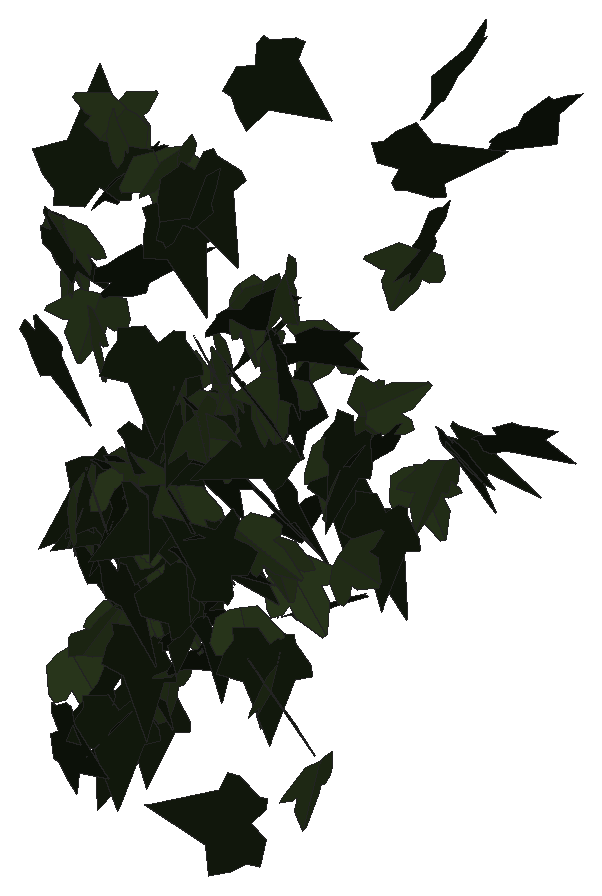
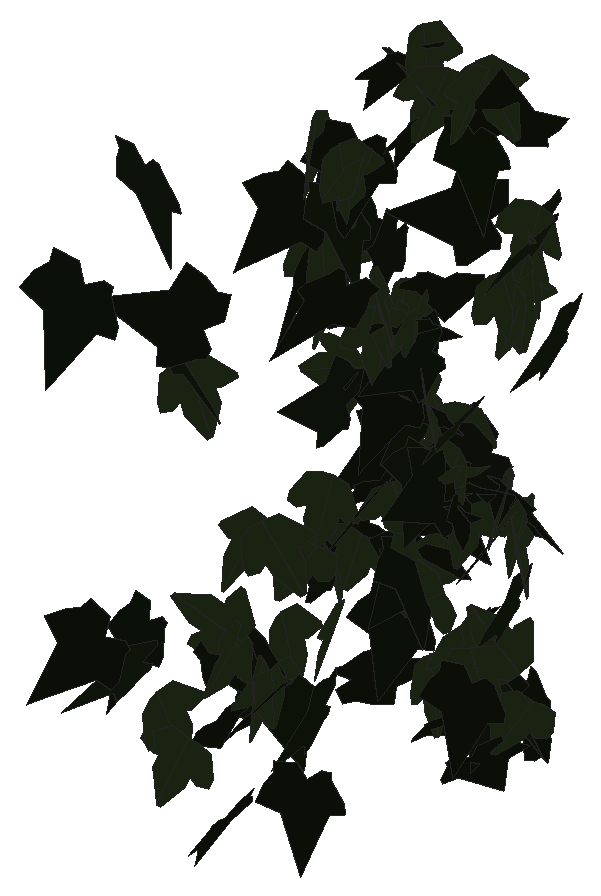
# SketchUp Ruby script. Lengths in inches.
U = 1.inch
M = Sketchup.active_model
def pt(a) = Geom::Point3d.new(a.map { |v| v * U })
def face(e, loops, mat)
  f = e.add_face(loops[0].map { |a| pt(a) })
  loops[1..].each { |l| e.add_face(l.map { |a| pt(a) }).erase! }
  f.material = f.back_material = mat if mat
  f
end
# faces: each face lists its corners as indices into pts; further lists are holes
def faces(e, pts, list, mat = nil) = list.each { |f| face(e, (f[0].is_a?(Array) ? f : [f]).map { |l| l.map { |i| pts[i] } }, mat) }
# xy, xz, yz: faces in a plane at the given z, y or x. An outline is a flat list of corners, or four numbers for a rectangle; further outlines are holes
def ring(l) = l.size == 4 ? [[l[0], l[1]], [l[2], l[1]], [l[2], l[3]], [l[0], l[3]]] : l.each_slice(2).to_a
def flat(e, list, mat, &to3) = list.each { |f| face(e, (f[0].is_a?(Array) ? f : [f]).map { |l| ring(l).map { |u, v| to3.(u, v) } }, mat) }
def xy(e, z, list, mat = nil) = flat(e, list, mat) { |x, y| [x, y, z] }
def xz(e, y, list, mat = nil) = flat(e, list, mat) { |x, z| [x, y, z] }
def yz(e, x, list, mat = nil) = flat(e, list, mat) { |y, z| [x, y, z] }
def lines(e, pts, list) = list.each { |a, b| e.add_line(pt(pts[a]), pt(pts[b])) }
# prism: a flat outline (further loops are holes) pulled along v
def prism(e, loops, v, mat = nil)
  f = face(e, loops, mat); d = Geom::Vector3d.new(v.map { |x| x * U })
  f.pushpull(f.normal.samedirection?(d) ? d.length : -d.length)
end
def box(e, o, s, mat = nil) = prism(e, [[o, [o[0] + s[0], o[1], o[2]], [o[0] + s[0], o[1] + s[1], o[2]], [o[0], o[1] + s[1], o[2]]]], [0, 0, s[2]], mat)
def at(x, y, z, deg = 0) = Geom::Transformation.translation(pt([x, y, z])) * Geom::Transformation.rotation(ORIGIN, Z_AXIS, deg.degrees)
def axes(o, x, y, z) = Geom::Transformation.new([*x, 0, *y, 0, *z, 0, *pt(o).to_a, 1])
def part(name) = M.definitions.add(name)
# library, detail: a bought-in or finely detailed component or shape, given as its bounding box
def library(name, o, s) = part(name).tap { |d| box(d.entities, o, s) }
def detail(e, o, s) = box(e.add_group.entities, o, s)
def put(e, d, t, mat = nil) = e.add_instance(d, t).tap { |i| i.material = mat if mat }
def group(e, t, mat = nil) = e.add_group.tap { |g| g.transformation = t; g.material = mat if mat }.entities
root = M.entities
M.materials.add("efeu1").color = [18, 25, 13]
M.materials.add("efeu2").color = [43, 57, 29]
c1 = part("ivyleaf_10")
p = [[0,0.5,-0.03],[-0.0625,2.02,-0.43],[-0.19,2.01,-0.46],[-0.54,1.05,-0.29],[-0.52,0.625,-0.18],[-0.83,0.76,-0.28],
  [-1.16,0.64,-0.33],[-1.15,0.33,-0.24],[-0.77,-0.39,0.02],[-0.3,-0.51,0.16],[0.04,-0.48,0.23],[-0.02,2.01,-0.4375],
  [-0.06,2.01,-0.43],[0.04,-0.49,0.23],[0.67,-0.49,0.14],[1.38,0.36,-0.2],[1.375,0.51,-0.24],[0.81,0.65,-0.19],
  [0.62,0.59,-0.15],[0.6,1.09,-0.28],[0.5,1.23,-0.31]]
faces(c1.entities,p,[[0,1,2,3,4,5,6,7,8,9,10],[11,12,0,13,14,15,16,17,18,19,20]],"efeu2")
c2 = part("ivyleaf_9")
p = [[1.54,2.16,1.25],[1.36,2.04,1.19],[-0.21,0.99,0.68],[-0.71,1.11,0.82],[-0.85,0.86,0.67],[-0.8,0.17,0.21],
  [-0.9,-0.01,0.1],[-0.67,-0.16,-0.02],[-0.08,-0.08,-0.05],[-0.03,-0.6,-0.4],[0.65,-0.88,-0.66],[0.83,-0.6,-0.49],
  [1.29,-0.42,-0.43],[1.8125,-0.07,-0.26],[1.21,0.44,0.15]]
faces(c2.entities,p,[[0,1,2,3,4,5,6,7,8,9,10,11,12,13,14]],"efeu1")
put(root,c1,axes([615.85,124.16,302.23],[-0.0433,-1.22848,-0.26768],[-0.03456,0.2689,-1.22849],[1.25683,-0.03493,-0.043]))
put(root,c2,axes([618.39,123.99,286.45],[-0.35286,0.28688,1.16377],[-0.96507,0.65147,-0.45321],[-0.71085,-1.02687,0.0376]))
put(root,c2,axes([610.3,124.6,276.83],[0.56426,-0.2794,-1.05982],[1.09365,0.22208,0.52372],[0.07223,-1.17995,0.34953]))
put(root,c2,axes([618.38,125.02,275.8125],[-0.40978,-0.84585,-0.82752],[-0.32548,-0.76138,0.93943],[-1.13768,0.52249,0.0293]))
put(root,c1,axes([619.14,124.4,287.95],[-0.46391,0.13468,-1.0838],[1.04968,-0.27011,-0.48287],[-0.30152,-1.14755,-0.01354]))
put(root,c2,axes([609.46,124.39,292.78],[0.94353,-0.81452,-0.23788],[-0.16787,0.16953,-1.24634],[0.83177,0.95818,0.0183]))
put(root,c2,axes([615.51,124.66,299.51],[0.32492,-1.16376,-0.32096],[-0.04184,0.32133,-1.20745],[1.20648,0.32456,0.04457]))
put(root,c2,axes([616.59,123.66,300.24],[0.126,0.73833,0.99377],[-0.65835,0.88592,-0.57473],[-1.04847,-0.46755,0.48031]))
put(root,c2,axes([612.74,124.89,283.93],[0.66806,-0.98934,0.14029],[0.0638,-0.12619,-1.19365],[0.9972,0.67086,-0.01762]))
put(root,c2,axes([612.64,124.95,278.25],[-0.6587,-0.72747,-0.60798],[0.50762,0.35464,-0.97431],[0.80073,-0.82326,0.11753]))
put(root,c2,axes([616.375,124.68,301.65],[0.15711,-1.07885,-0.60291],[0.15114,0.61997,-1.07],[1.22661,0.06179,0.20907]))
put(root,c1,axes([616.58,124.44,291.76],[0.01717,-1.10472,-0.47812],[0.09681,0.47789,-1.1007],[1.19984,-0.02275,0.09566]))
put(root,c2,axes([612.21,124.39,300],[-1.27822,-0.28751,0.55165],[0.53934,0.116,1.31015],[-0.31,1.38734,0.00478]))
put(root,c2,axes([614.18,125.2,293.59],[-0.5532,-0.9828,-0.49121],[0.43229,0.31091,-1.1089],[1.0101,-0.67131,0.20556]))
put(root,c2,axes([618.07,125.27,293.4],[0.61137,-0.79804,0.71074],[0.49994,-0.51012,-1.00281],[0.9445,0.78658,0.07074]))
put(root,c1,axes([615.65,124.88,288.05],[-1.10346,-0.11334,-0.39142],[0.40573,-0.20025,-1.08581],[0.03798,-1.15358,0.22694]))
put(root,c2,axes([610.11,124.48,297.16],[1.00556,-0.444,-0.55518],[-0.37168,0.49145,-1.06623],[0.60598,1.0382,0.26729]))
put(root,c2,axes([619.625,125.77,294.31],[0.03489,-0.46323,1.1072],[0.19537,-1.0907,-0.46249],[1.18419,0.19359,0.04368]))
put(root,c1,axes([614.625,124.91,301.27],[-0.93457,-0.71839,-0.39001],[0.48277,-0.00703,-1.1439],[0.65964,-1.01266,0.28462]))
put(root,c1,axes([610.46,124.86,297.15],[-1.19553,0.13285,-0.14595],[0.13754,-0.08177,-1.2011],[-0.14154,-1.20163,0.0656]))
put(root,c1,axes([612.5,125.16,302.36],[-0.94227,-0.36306,0.71281],[-0.60761,-0.39157,-1.00264],[0.52032,-1.11474,0.12003]))
put(root,c1,axes([610.3,125.01,296.03],[0.93697,-0.7882,-0.09332],[0.07276,0.22907,-1.20421],[0.79036,0.91332,0.22149]))
put(root,c2,axes([618.75,124.43,297.07],[0.38161,1.15016,-0.07246],[-0.03535,-0.06461,-1.21174],[-1.1519,0.38302,0.01318]))
put(root,c2,axes([614.35,125.82,286.55],[-0.94205,-0.44896,0.52127],[-0.34243,-0.46059,-1.01555],[0.59667,-0.97316,0.24017]))
put(root,c1,axes([611.38,125.28,294.25],[-0.80375,-0.85619,0.34099],[-0.16184,-0.31429,-1.17063],[0.90727,-0.81456,0.09326]))
put(root,c2,axes([616.9375,124.66,294.2],[0.92576,-0.09633,-0.76545],[-0.7489,0.17504,-0.92776],[0.18534,1.18841,0.0746]))
put(root,c2,axes([612.93,124.46,296.2],[0.64303,0.07724,1.11184],[0.91532,0.69576,-0.57771],[-0.63588,1.07962,0.29276]))
put(root,c2,axes([615.18,125.35,287.5625],[0.97691,-0.6502,-0.05486],[-0.05628,0.01444,-1.17335],[0.65008,0.97834,-0.01915]))
put(root,c2,axes([615.5625,125.41,284.03],[-0.99219,0.31067,0.52272],[-0.48685,0.1935,-1.0391],[-0.36433,-1.10464,-0.03501]))
put(root,c1,axes([610.91,125.32,293.71],[-0.95358,0.71123,-0.27459],[0.19567,-0.19668,-1.18895],[-0.73686,-0.97264,0.03963]))
put(root,c2,axes([616.18,124.86,286.23],[1.07533,0.33696,0.32128],[0.28206,0.17182,-1.12429],[-0.37041,1.10907,0.07657]))
put(root,c1,axes([617.2,125.3,290.77],[0.35485,0.16747,-1.12453],[-1.08733,0.39415,-0.28441],[0.33215,1.11137,0.27032]))
put(root,c2,axes([614.625,125.91,288.39],[-0.99857,-0.35101,-0.50364],[0.48678,0.13317,-1.05797],[0.37403,-1.11043,0.03232]))
put(root,c1,axes([618.46,125.64,297.09],[-0.17537,-1.20364,0.01617],[-0.01059,-0.0148,-1.21632],[1.2037,-0.17549,-0.00835]))
put(root,c1,axes([613.24,125.43,288.28],[-1.17577,-0.05594,0.1598],[-0.15831,-0.03425,-1.1768],[0.06003,-1.18609,0.02644]))
put(root,c1,axes([618.05,125.38,296.77],[-0.10181,1.22145,0.02751],[-0.00084,0.02753,-1.22568],[-1.22176,-0.1018,-0.00145]))
put(root,c2,axes([619.01,126.18,291.05],[-1.06825,-0.18471,0.47145],[-0.42037,-0.29007,-1.06616],[0.28226,-1.13105,0.19644]))
put(root,c2,axes([615.42,126.2,291.61],[-0.84454,-0.82833,-0.18309],[0.19174,0.06528,-1.17978],[0.82637,-0.86169,0.08662]))
put(root,c1,axes([619,125.65,281.72],[0.39826,-1.13674,-0.19511],[-0.06503,0.18395,-1.20449],[1.15153,0.40353,-0.00054]))
put(root,c2,axes([618.59,126.06,280.9],[0.65392,-0.73237,0.65307],[0.42924,-0.49224,-0.98181],[0.8824,0.78219,-0.00638]))
put(root,c2,axes([611.18,125.97,286.51],[-1.17568,0.08003,-0.01328],[0.01323,-0.00121,-1.1784],[-0.08004,-1.17575,0.00031]))
put(root,c1,axes([619.33,125.78,293.39],[-0.91338,-0.76601,0.12842],[-0.08853,-0.09427,-1.19197],[0.77163,-0.91753,0.01525]))
put(root,c2,axes([612.21,124.9,277.19],[0.1203,1.0288,0.50547],[0.01188,0.5071,-1.03495],[-1.14621,0.11323,0.04233]))
put(root,c1,axes([613.81,125.73,286.625],[-1.09389,0.17325,-0.34606],[0.3328,-0.10845,-1.10628],[-0.19752,-1.14219,0.05255]))
put(root,c2,axes([611.64,125.73,278.56],[-0.87687,0.74677,0.00919],[-0.02995,-0.02101,-1.15122],[-0.74622,-0.87667,0.03541]))
put(root,c1,axes([619.69,125.57,297.97],[0.33165,-1.04789,-0.51734],[0.1186,0.56517,-1.06875],[1.1626,0.24127,0.2566]))
put(root,c2,axes([612.49,126.45,280.24],[0.11928,-1.17597,0.11698],[0.03769,-0.11373,-1.18172],[1.18117,0.12239,0.02589]))
put(root,c1,axes([612.58,125.29,302.2],[-0.06167,1.04487,0.65522],[-0.16441,0.64321,-1.04121],[-1.22231,-0.13923,0.10699]))
put(root,c2,axes([618.29,126.42,282.27],[-0.27917,-1.11605,-0.265],[0.13904,0.2378,-1.14798],[1.13863,-0.30267,0.07521]))
put(root,c2,axes([612.02,126.66,286.39],[-0.28964,0.22164,-1.12381],[0.70661,-0.87777,-0.35523],[-0.90154,-0.75918,0.08263]))
put(root,c2,axes([612.65,125.49,300.03],[-0.17854,1.21356,0.01299],[-0.00308,0.01267,-1.22662],[-1.21362,-0.17856,0.0012]))
put(root,c1,axes([610.99,125.75,286.46],[-0.69431,0.94249,0.13022],[-0.04889,0.12565,-1.1701],[-0.95018,-0.69515,-0.03495]))
put(root,c2,axes([612.03,126.6,285.96],[-1.06601,-0.31545,0.39903],[-0.38314,-0.11152,-1.1117],[0.33458,-1.13277,-0.00168]))
put(root,c1,axes([614.77,126.17,292.38],[-0.17309,1.14607,-0.2796],[0.02214,-0.27939,-1.15891],[-1.17947,-0.17343,0.01927]))
put(root,c1,axes([610.27,125.7,285.76],[-0.26267,1.10482,0.38543],[-0.2522,0.33228,-1.12435],[-1.14262,-0.32732,0.15957]))
put(root,c2,axes([615.42,126.88,281.61],[0.27259,-0.89059,0.71161],[0.22192,-0.67621,-0.93131],[1.11816,0.35132,0.01136]))
put(root,c2,axes([618.69,125.63,295.19],[-0.26247,1.15079,0.26935],[-0.22749,0.22156,-1.16829],[-1.15979,-0.3039,0.1682]))
put(root,c1,axes([610.05,126.25,285.23],[0.51511,-1.02657,-0.21563],[-0.07154,0.20529,-1.14823],[1.04653,0.51932,0.02765]))
put(root,c1,axes([614.04,126.4,289.92],[0.59096,-1.03315,-0.04774],[0.04694,0.08172,-1.18745],[1.03318,0.58723,0.08126]))
put(root,c1,axes([611.89,126.27,286.84],[0.80807,0.82571,0.10135],[0.09115,0.05255,-1.15498],[-0.8269,0.8127,-0.02828]))
put(root,c1,axes([616.26,126.29,291.53],[-1.03614,-0.54972,0.0504],[-0.04306,-0.02636,-1.17293],[0.55034,-1.03703,0.0031]))
put(root,c1,axes([610.56,126.22,279.82],[-0.22579,-1.13162,0.41676],[0.2857,0.36173,1.137],[-1.1716,0.3063,0.19694]))
put(root,c2,axes([614.13,126.18,291.12],[1.14412,-0.26341,0.18836],[0.17791,-0.06662,-1.17379],[0.27058,1.1576,-0.02469]))
put(root,c1,axes([620.27,126.57,277.85],[0.03457,-1.20831,0.06088],[0.02536,-0.06017,-1.20858],[1.20958,0.0358,0.0236]))
put(root,c2,axes([615.55,127.06,285.77],[-0.50957,-1.0459,0.04124],[0.02368,-0.05737,-1.1625],[1.04644,-0.508,0.04639]))
put(root,c2,axes([611.74,125.87,287.65],[1.16221,0.16587,0.15595],[0.12804,0.19452,-1.16118],[-0.18825,1.15638,0.17296]))
put(root,c2,axes([615.74,126.01,289.09],[1.0395,0.39973,-0.36048],[-0.34035,-0.11925,-1.11366],[-0.41701,1.09375,0.01033]))
put(root,c1,axes([616.58,126.26,292.37],[-0.78411,0.27745,0.8565],[-0.83418,0.20341,-0.82956],[-0.33871,-1.14326,0.06026]))
put(root,c2,axes([612.52,126.61,288.82],[0.70665,-0.92144,-0.233],[0.02607,0.30903,-1.14303],[0.95008,0.67687,0.20467]))
put(root,c2,axes([612.9,127.15,285.22],[-0.98688,-0.60213,-0.04896],[0.03746,0.0326,-1.15603],[0.60295,-0.98755,-0.00831]))
put(root,c2,axes([614.01,126.96,283.36],[-0.76524,-0.65826,-0.57461],[0.44937,0.35858,-1.00924],[0.74937,-0.88724,0.01843]))
put(root,c1,axes([614.1,127.01,282.81],[0.50968,0.62714,0.84354],[-0.53216,-0.6545,0.80813],[0.90646,-0.73686,0.00013]))
put(root,c1,axes([616.84,126.69,282.59],[1.05419,0.29448,0.43772],[0.41267,0.14904,-1.09413],[-0.32866,1.13168,0.0302]))
put(root,c1,axes([612.7,126.66,287.31],[-1.01841,0.50851,-0.21546],[0.16754,-0.14621,-1.13697],[-0.52625,-1.03063,0.05499]))
put(root,c2,axes([617.49,126.86,288.1],[0.87292,-0.6159,0.48853],[0.44101,-0.22067,-1.06621],[0.65077,0.97568,0.06724]))
put(root,c1,axes([612.04,126.6,285.8125],[-1.17841,0.07851,0.02241],[-0.02232,0.00209,-1.18102],[-0.07853,-1.17862,-0.0006]))
put(root,c2,axes([610.57,127.21,284.96],[0.4097,-1.08647,0.0558],[0.01224,-0.05502,-1.16113],[1.08783,0.40981,-0.00795]))
put(root,c1,axes([618.21,126.16,292.44],[-0.25558,0.90949,0.72909],[-0.26183,0.68254,-0.94321],[-1.13586,-0.36198,0.05336]))
put(root,c1,axes([616.28,126.39,293],[0.417,-0.5299,-0.96676],[-0.61362,0.74714,-0.67421],[0.9159,0.74182,-0.01154]))
put(root,c2,axes([614.84,125.9,282.27],[0.39429,0.9439,0.60512],[0.18717,0.57703,-1.02204],[-1.10548,0.43436,0.04278]))
put(root,c2,axes([611.04,127.51,276.3],[-0.50718,-1.03041,0.02613],[-0.04921,-0.00489,-1.1477],[1.02957,-0.50783,-0.04198]))
put(root,c1,axes([609.33,126.64,278.43],[0.76272,0.62275,0.63122],[0.481,0.40889,-0.9846],[-0.74491,0.90166,0.01053]))
put(root,c2,axes([612.14,127.53,277.61],[-0.17152,-1.13794,0.04407],[0.12183,-0.06265,-1.14346],[1.13225,-0.16564,0.12971]))
put(root,c2,axes([619.84,126.25,295.27],[0.90278,0.72377,0.29673],[0.19654,0.22871,-1.15584],[-0.75714,0.92236,0.05377]))
put(root,c2,axes([609.51,127.01,283.04],[0.84628,-0.74689,-0.2137],[-0.17691,0.12243,-1.12846],[0.75645,0.86422,-0.02483]))
put(root,c1,axes([614.87,127.1,285.54],[0.61837,0.9457,-0.28185],[-0.2665,-0.16021,-1.12226],[-0.95014,0.66042,0.13134]))
put(root,c2,axes([611.46,127.36,279.59],[0.6509,-0.93631,0.19432],[0.12987,-0.14634,-1.1401],[0.94741,0.66333,0.02277]))
put(root,c1,axes([613.125,127.18,278.91],[-0.17283,-1.14447,-0.10702],[0.00435,0.10757,-1.15738],[1.14945,-0.17249,-0.01171]))
put(root,c1,axes([612.91,127.24,282.08],[0.67211,-0.07652,0.94431],[0.94515,0.13391,-0.66186],[-0.06526,1.15131,0.13975]))
put(root,c2,axes([619.49,126.51,292.77],[0.3025,-0.0139,-1.14852],[-0.94126,0.67767,-0.25612],[0.65827,0.97538,0.16157]))
put(root,c1,axes([611.65,127.5,281.09],[0.18157,1.07975,-0.35314],[-0.07956,-0.34466,-1.09473],[-1.13325,0.1972,0.02028]))
put(root,c2,axes([614.25,126.99,283.15],[-0.15078,1.1485,-0.09498],[0.02592,-0.09239,-1.15827],[-1.15213,-0.15238,-0.01363]))
put(root,c2,axes([615.51,127.125,285.47],[0.71558,-0.63693,-0.66418],[-0.2816,0.64944,-0.92618],[0.87609,0.72899,0.2448]))
put(root,c2,axes([613.57,126.66,286.66],[0.3276,1.03972,0.40292],[-0.04668,0.43237,-1.07776],[-1.11409,0.28762,0.16364]))
put(root,c2,axes([614.7,127.02,280.73],[0.35946,1.10542,0.12641],[-0.00788,0.13537,-1.16136],[-1.1126,0.35618,0.04906]))
put(root,c1,axes([610.78,127.68,280.38],[0.99781,0.50477,-0.25471],[-0.36368,0.17741,-1.07311],[-0.43291,1.01441,0.31442]))
put(root,c2,axes([612.69,127.08,286.45],[0.44996,0.54735,0.92162],[0.33033,0.88007,-0.68395],[-1.01973,0.52661,0.1851]))
put(root,c1,axes([617.22,128.13,285.23],[-1.1556,-0.0944,-0.0961],[0.09597,0.00549,-1.15945],[0.09453,-1.15958,0.00233]))
put(root,c2,axes([610.5625,128.27,279.65],[0.29604,1.10278,0.04301],[-0.00297,0.04532,-1.14173],[-1.10362,0.29569,0.01461]))
put(root,c1,axes([616.95,129.46,283.3],[0.72222,0.69786,0.59073],[0.44214,0.39235,-1.00406],[-0.8003,0.84654,-0.02161]))
put(root,c1,axes([618.67,130.42,284.09],[0.18339,0.74373,0.8887],[-0.23426,0.90498,-0.70901],[-1.13493,-0.06662,0.28995]))
put(root,c2,axes([615.49,133.12,280.13],[-0.00783,1.13626,-0.24426],[-0.47012,-0.22648,-1.03851],[-1.06289,0.09181,0.46114]))
put(root,c1,axes([617.13,136.0625,293.42],[-0.77412,-0.79521,0.40229],[-0.29008,-0.27901,-1.10971],[0.84264,-0.82659,-0.01244]))
put(root,c2,axes([617.97,136.04,294.62],[-0.88649,0.77661,-0.13606],[0.09509,-0.09793,-1.1785],[-0.78268,-0.8915,0.01093]))
put(root,c2,axes([611,136.11,282.15],[0.97141,-0.67413,-0.28389],[-0.23442,0.16013,-1.18241],[0.69289,0.9993,-0.00204]))
put(root,c2,axes([610.5,135.59,299.11],[0.26834,-0.42782,-1.15544],[-0.16132,1.16015,-0.46702],[1.2215,0.2472,0.19216]))
put(root,c1,axes([613.11,136.52,288.46],[-0.86344,-0.46477,0.66975],[-0.52355,-0.43167,-0.97451],[0.62489,-1.00387,0.10896]))
put(root,c2,axes([613.75,136.85,284.58],[-1.00688,-0.03935,-0.6563],[0.65498,0.04446,-1.00753],[0.05723,-1.20107,-0.0158]))
put(root,c2,axes([618.82,136.4,301.375],[-0.50228,1.23046,0.50187],[-0.21639,0.45363,-1.32875],[-1.31113,-0.54624,0.02704]))
put(root,c2,axes([612.64,137.84,282.19],[0.11404,-1.1227,0.22085],[0.0691,-0.21478,-1.12754],[1.14213,0.12509,0.04616]))
put(root,c1,axes([612.41,137.31,283.32],[0.27327,1.14546,-0.19753],[-0.08007,-0.18388,-1.1771],[-1.15961,0.28263,0.03473]))
put(root,c1,axes([609.86,136.84,286.53],[-0.49926,0.95392,0.44885],[-0.18152,0.41144,-1.07632],[-1.0385,-0.53052,-0.02766]))
put(root,c2,axes([614.33,137.9375,281.1875],[-0.00031,-1.1861,0.07634],[-0.01511,-0.07633,-1.18601],[1.18846,-0.00128,-0.01506]))
put(root,c1,axes([613.11,136.88,283],[0.1855,-0.83102,-0.84],[-0.10974,0.83449,-0.84981],[1.1765,0.20887,0.05318]))
put(root,c2,axes([614.28,137.72,284.34],[-0.50638,0.75103,-0.72225],[0.22583,-0.70483,-0.89125],[-1.0172,-0.53035,0.16168]))
put(root,c2,axes([615.88,137.07,296.27],[0.45442,0.02056,1.2266],[1.22175,0.1107,-0.45447],[-0.11093,1.30338,0.01925]))
put(root,c2,axes([610.31,137.92,280.05],[0.24852,1.10795,-0.11448],[-0.09116,-0.09667,-1.13347],[-1.11011,0.25598,0.06745]))
put(root,c1,axes([613.67,138.14,285.17],[-0.49412,-0.48923,0.92476],[0.68205,0.62487,0.69501],[-0.79331,0.84195,0.02154]))
put(root,c1,axes([613.22,138.17,284.81],[-0.02785,-0.61059,-0.9805],[0.16718,0.96833,-0.60776],[1.14292,-0.15652,0.06501]))
put(root,c2,axes([616.92,138.7,284.55],[1.08687,0.01255,-0.51831],[-0.51846,0.01986,-1.08669],[-0.00278,1.20397,0.02333]))
put(root,c1,axes([615.14,139.95,282.34],[-0.18049,-1.11285,0.38624],[-0.00356,-0.39023,-1.12601],[1.17796,-0.1717,0.05578]))
put(root,c2,axes([612.16,140.24,278.98],[0.40279,-1.07979,-0.23813],[-0.06501,0.22987,-1.15231],[1.10382,0.40756,0.01903]))
put(root,c2,axes([616.12,140.12,283.89],[1.06652,-0.48671,-0.23478],[-0.00781,0.50552,-1.08345],[0.54032,0.96801,0.44776]))
put(root,c2,axes([619.05,139.71,297.92],[0.38028,1.3043,0.32834],[0.09318,0.31485,-1.35861],[-1.34176,0.39153,-0.00129]))
put(root,c1,axes([613.8,140.49,281.28],[1.06587,0.20437,0.47791],[0.36989,0.46776,-1.025],[-0.36516,1.07036,0.35669]))
put(root,c2,axes([617.58,140.45,284.48],[1.01513,0.56622,0.29144],[0.18531,0.26204,-1.15457],[-0.60926,1.02311,0.13441]))
